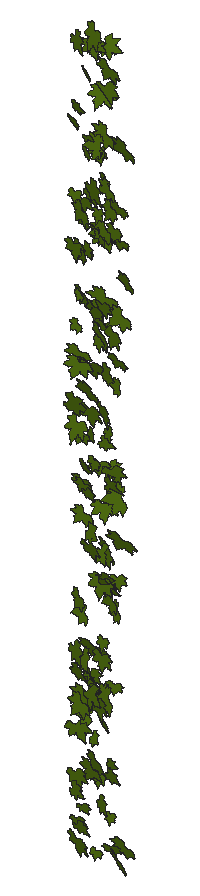
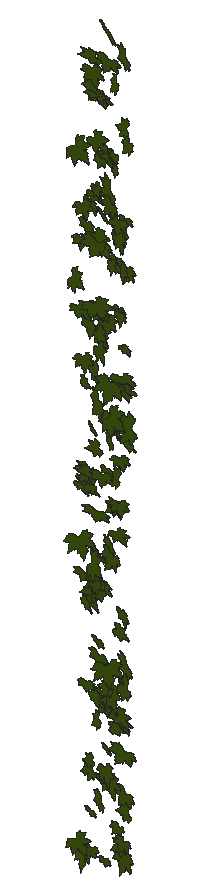
# SketchUp Ruby script. Lengths in inches.
U = 1.inch
M = Sketchup.active_model
def pt(a) = Geom::Point3d.new(a.map { |v| v * U })
def face(e, loops, mat)
  f = e.add_face(loops[0].map { |a| pt(a) })
  loops[1..].each { |l| e.add_face(l.map { |a| pt(a) }).erase! }
  f.material = f.back_material = mat if mat
  f
end
# faces: each face lists its corners as indices into pts; further lists are holes
def faces(e, pts, list, mat = nil) = list.each { |f| face(e, (f[0].is_a?(Array) ? f : [f]).map { |l| l.map { |i| pts[i] } }, mat) }
# xy, xz, yz: faces in a plane at the given z, y or x. An outline is a flat list of corners, or four numbers for a rectangle; further outlines are holes
def ring(l) = l.size == 4 ? [[l[0], l[1]], [l[2], l[1]], [l[2], l[3]], [l[0], l[3]]] : l.each_slice(2).to_a
def flat(e, list, mat, &to3) = list.each { |f| face(e, (f[0].is_a?(Array) ? f : [f]).map { |l| ring(l).map { |u, v| to3.(u, v) } }, mat) }
def xy(e, z, list, mat = nil) = flat(e, list, mat) { |x, y| [x, y, z] }
def xz(e, y, list, mat = nil) = flat(e, list, mat) { |x, z| [x, y, z] }
def yz(e, x, list, mat = nil) = flat(e, list, mat) { |y, z| [x, y, z] }
def lines(e, pts, list) = list.each { |a, b| e.add_line(pt(pts[a]), pt(pts[b])) }
# prism: a flat outline (further loops are holes) pulled along v
def prism(e, loops, v, mat = nil)
  f = face(e, loops, mat); d = Geom::Vector3d.new(v.map { |x| x * U })
  f.pushpull(f.normal.samedirection?(d) ? d.length : -d.length)
end
def box(e, o, s, mat = nil) = prism(e, [[o, [o[0] + s[0], o[1], o[2]], [o[0] + s[0], o[1] + s[1], o[2]], [o[0], o[1] + s[1], o[2]]]], [0, 0, s[2]], mat)
def at(x, y, z, deg = 0) = Geom::Transformation.translation(pt([x, y, z])) * Geom::Transformation.rotation(ORIGIN, Z_AXIS, deg.degrees)
def axes(o, x, y, z) = Geom::Transformation.new([*x, 0, *y, 0, *z, 0, *pt(o).to_a, 1])
def part(name) = M.definitions.add(name)
# library, detail: a bought-in or finely detailed component or shape, given as its bounding box
def library(name, o, s) = part(name).tap { |d| box(d.entities, o, s) }
def detail(e, o, s) = box(e.add_group.entities, o, s)
def put(e, d, t, mat = nil) = e.add_instance(d, t).tap { |i| i.material = mat if mat }
def group(e, t, mat = nil) = e.add_group.tap { |g| g.transformation = t; g.material = mat if mat }.entities
root = M.entities
M.materials.add("[Vegetation Blur 03]").color = [83, 114, 18]
c1 = part("ivy")
xy(c1.entities,0,[[0.782,0,0.786,0,0.787,0.005,0.789,0.009,0.821,0.072,0.875,0.147,1.001,0.272,1.073,0.331,1.137,0.363,1.178,0.379,1.223,0.384,1.272,0.383,1.311,0.374,1.36,0.355,1.399,0.334,1.491,0.285,1.541,0.244,1.583,0.199,1.617,0.15,1.64,0.128,1.662,0.115,1.717,0.105,1.745,0.093,1.784,0.054,1.819,0.057,1.854,0.064,1.882,0.075,1.896,0.074,1.91,0.071,1.937,0.063,1.964,0.053,1.99,0.038,2.016,0.015,2.034,0.002,2.04,0,2.038,0.003,2.036,0.007,2.033,0.038,2.036,0.068,2.045,0.1,2.055,0.116,2.064,0.123,2.077,0.129,2.088,0.129,2.106,0.132,2.118,0.13,2.179,0.132,2.207,0.133,2.225,0.133,2.242,0.138,2.22,0.162,2.207,0.186,2.206,0.213,2.212,0.236,2.228,0.262,2.247,0.274,2.298,0.283,2.355,0.294,2.37,0.296,2.376,0.295,2.377,0.3,2.377,0.303,2.385,0.329,2.411,0.37,2.426,0.392,2.449,0.407,2.511,0.426,2.561,0.444,2.619,0.466,2.589,0.469,2.561,0.476,2.501,0.5,2.449,0.516,2.424,0.523,2.401,0.535,2.377,0.556,2.372,0.568,2.36,0.575,2.268,0.586,2.225,0.592,2.207,0.599,2.194,0.61,2.143,0.65,2.13,0.664,2.122,0.682,2.123,0.7,2.13,0.719,2.148,0.75,2.17,0.781,2.195,0.807,2.221,0.828,2.284,0.874,2.291,0.88,2.288,0.887,2.276,0.9,2.267,0.916,2.265,0.933,2.273,0.967,2.292,1.002,2.313,1.03,2.334,1.054,2.348,1.067,2.358,1.074,2.363,1.076,2.362,1.081,2.35,1.094,2.347,1.11,2.35,1.143,2.359,1.18,2.385,1.254,2.415,1.324,2.448,1.393,2.45,1.4,2.446,1.398,2.44,1.394,2.427,1.383,2.402,1.36,2.376,1.339,2.345,1.324,2.305,1.309,2.282,1.303,2.273,1.306,2.245,1.294,2.212,1.287,2.187,1.291,2.163,1.301,2.142,1.316,2.134,1.327,2.124,1.325,2.09,1.292,2.053,1.259,2.014,1.234,1.973,1.215,1.954,1.21,1.931,1.208,1.909,1.212,1.893,1.22,1.879,1.233,1.872,1.248,1.867,1.281,1.864,1.319,1.821,1.258,1.773,1.197,1.726,1.141,1.698,1.121,1.679,1.116,1.666,1.117,1.647,1.122,1.632,1.129,1.62,1.141,1.617,1.154,1.617,1.219,1.621,1.254,1.623,1.268,1.623,1.281,1.618,1.314,1.606,1.346,1.603,1.375,1.607,1.403,1.603,1.467,1.599,1.499,1.605,1.525,1.614,1.552,1.629,1.577,1.635,1.589,1.629,1.587,1.618,1.582,1.596,1.566,1.581,1.556,1.568,1.552,1.557,1.55,1.545,1.553,1.531,1.562,1.522,1.572,1.504,1.591,1.486,1.611,1.474,1.631,1.457,1.666,1.455,1.684,1.457,1.698,1.452,1.715,1.444,1.728,1.424,1.754,1.419,1.772,1.423,1.786,1.434,1.819,1.444,1.848,1.446,1.855,1.44,1.861,1.43,1.867,1.386,1.904,1.349,1.948,1.326,1.973,1.31,1.995,1.288,2.048,1.284,2.153,1.287,2.254,1.284,2.255,1.282,2.253,1.278,2.247,1.274,2.237,1.266,2.216,1.226,2.125,1.208,2.076,1.184,2.033,1.155,1.984,1.135,1.942,1.111,1.899,1.083,1.861,1.053,1.85,1.059,1.83,1.061,1.809,1.056,1.79,1.049,1.767,1.04,1.749,1.018,1.733,0.994,1.726,0.942,1.734,0.95,1.6875,0.944,1.645,0.932,1.608,0.911,1.585,0.881,1.58,0.854,1.582,0.828,1.588,0.785,1.618,0.773,1.625,0.775,1.614,0.779,1.598,0.796,1.502,0.818,1.402,0.861,1.283,0.882,1.224,0.894,1.174,0.892,1.148,0.886,1.123,0.881,1.107,0.872,1.099,0.849,1.094,0.818,1.092,0.789,1.098,0.762,1.107,0.753,1.113,0.721,1.139,0.698,1.163,0.678,1.194,0.665,1.224,0.628,1.28,0.612,1.312,0.606,1.327,0.606,1.314,0.599,1.282,0.594,1.267,0.581,1.256,0.544,1.245,0.512,1.244,0.473,1.249,0.444,1.256,0.382,1.288,0.339,1.306,0.324,1.316,0.317,1.324,0.309,1.326,0.27,1.314,0.227,1.313,0.185,1.3125,0.152,1.317,0.122,1.328,0.092,1.345,0.073,1.353,0.079,1.338,0.092,1.308,0.117,1.249,0.13,1.215,0.139,1.164,0.147,1.148,0.157,1.136,0.163,1.122,0.174,1.086,0.177,1.067,0.182,1.054,0.186,1.043,0.191,1.038,0.211,1.028,0.237,1.005,0.25,0.974,0.253,0.96,0.25,0.944,0.242,0.914,0.243,0.906,0.249,0.902,0.26,0.894,0.289,0.88,0.307,0.873,0.322,0.862,0.364,0.799,0.403,0.738,0.431,0.709,0.439,0.691,0.441,0.678,0.4375,0.66,0.428,0.645,0.394,0.623,0.303,0.594,0.255,0.581,0.214,0.577,0.179,0.573,0.173,0.568,0.175,0.561,0.167,0.55,0.141,0.523,0.113,0.503,0.077,0.49,0.045,0.486,0.026,0.485,0.019,0.486,0.011,0.483,0,0.471,0.014,0.467,0.044,0.455,0.058,0.447,0.07,0.438,0.097,0.411,0.125,0.394,0.158,0.377,0.174,0.366,0.182,0.359,0.185,0.361,0.242,0.331,0.253,0.316,0.258,0.303,0.262,0.283,0.274,0.278,0.308,0.274,0.341,0.252,0.366,0.226,0.366,0.222,0.37,0.22,0.38,0.221,0.395,0.221,0.425,0.216,0.45,0.207,0.465,0.192,0.473,0.178,0.484,0.15,0.489,0.116,0.483,0.089,0.468,0.058,0.45,0.035,0.435,0.018,0.429,0.011,0.434,0.012,0.438,0.014,0.469,0.019,0.542,0.016,0.581,0.015,0.612,0.027,0.68,0.055,0.696,0.057,0.712,0.052,0.73,0.045,0.741,0.036,0.766,0.014]])
put(root,c1,axes([131.39,173.8,39.79],[0.32765,-0.02489,0.01881],[0.02157,-0.07508,-0.26601],[-0.01455,-0.67173,0.02903]),"[Vegetation Blur 03]")
put(root,c1,axes([131.42,173.8,31.85],[0.50815,0.02983,-0.17456],[-0.21367,-0.02159,-0.41487],[0.01743,-1.13431,0.00331]),"[Vegetation Blur 03]")
put(root,c1,axes([131.75,173.8,33.24],[0.24945,-0.08617,-0.15972],[-0.19859,-0.02674,-0.20432],[-0.02483,-0.6519,0.02949]),"[Vegetation Blur 03]")
put(root,c1,axes([131.27,173.8,43.5625],[0.34754,-0.2147,0.09746],[0.13272,0.06991,-0.29103],[-0.08677,-0.75297,-0.05481]),"[Vegetation Blur 03]")
put(root,c1,axes([132.4375,173.8,30.04],[0.15268,0.21133,-0.48982],[-0.60568,0.18355,-0.11329],[-0.06257,-1.26109,-0.09857]),"[Vegetation Blur 03]")
put(root,c1,axes([131.4,173.8,31.3],[0.55742,0.02012,-0.13001],[-0.15728,-0.13301,-0.4524],[0.0271,-1.18554,0.04855]),"[Vegetation Blur 03]")
put(root,c1,axes([131.15,173.8,37.24],[0.58629,-0.17522,0.04019],[0.04988,0.00183,-0.48347],[-0.08478,-1.21072,-0.00655]),"[Vegetation Blur 03]")
put(root,c1,axes([131.63,173.8,27.5],[0.38921,0.02788,-0.11804],[-0.14492,0.01541,-0.31769],[0.01009,-0.85429,-0.00958]),"[Vegetation Blur 03]")
put(root,c1,axes([131.97,173.8,39.32],[0.36249,-0.1648,-0.3565],[-0.41016,0.32061,-0.3011],[-0.17026,-1.12322,-0.03364]),"[Vegetation Blur 03]")
put(root,c1,axes([131.62,173.8,25.16],[0.40951,0.01971,-0.10583],[-0.13003,0.06915,-0.33309],[-0.00105,-0.88123,-0.0285]),"[Vegetation Blur 03]")
put(root,c1,axes([131.39,173.8,7.37],[0.37849,-0.06704,0.09137],[0.11442,0.06293,-0.30843],[-0.02244,-0.80977,-0.03153]),"[Vegetation Blur 03]")
put(root,c1,axes([131.02,173.8,12.03],[0.53376,0.03726,0.21952],[0.269,0.00727,-0.43585],[0.01776,-1.22992,0.00407]),"[Vegetation Blur 03]")
put(root,c1,axes([131.98,173.8,14.45],[0.42826,-0.11256,-0.35023],[-0.42906,0.04831,-0.35189],[-0.05529,-1.24664,0.01798]),"[Vegetation Blur 03]")
put(root,c1,axes([131.08,173.8,28.28],[0.20202,-0.16973,0.51163],[0.63222,0.07532,-0.16235],[0.00985,-1.35325,-0.07321]),"[Vegetation Blur 03]")
put(root,c1,axes([132.31,173.8,18.72],[0.19822,-0.13225,-0.36337],[-0.44645,0.06503,-0.16594],[-0.0552,-1.0008,0.03723]),"[Vegetation Blur 03]")
put(root,c1,axes([131.39,173.8,8.5],[0.13655,-0.05783,0.35944],[0.43753,-0.10617,-0.1134],[-0.05764,-0.9429,-0.00928]),"[Vegetation Blur 03]")
put(root,c1,axes([131.75,173.8,14.03],[0.51915,-0.17766,-0.225],[-0.28069,-0.03421,-0.42714],[-0.06834,-1.20911,0.04515]),"[Vegetation Blur 03]")
put(root,c1,axes([131.17,173.8,9.74],[0.52125,-0.12471,0.19571],[0.23821,-0.0569,-0.42827],[-0.06661,-1.17932,-0.00003]),"[Vegetation Blur 03]")
put(root,c1,axes([131.91,173.8,23.69],[0.40363,-0.02669,-0.22372],[-0.27442,-0.04788,-0.32887],[0.00236,-1.00289,0.02165]),"[Vegetation Blur 03]")
put(root,c1,axes([131.85,173.8,25.06],[0.38167,-0.01698,-0.15187],[-0.18516,0.0606,-0.31101],[-0.02031,-0.87168,-0.01866]),"[Vegetation Blur 03]")
put(root,c1,axes([131.73,173.8,19.37],[0.45232,-0.27078,-0.13351],[-0.16346,0.04761,-0.38403],[-0.13176,-0.98864,0.01808]),"[Vegetation Blur 03]")
put(root,c1,axes([131.875,173.8,34.86],[0.28246,-0.12607,-0.06429],[-0.08477,-0.04633,-0.23378],[-0.05266,-0.60166,0.03147]),"[Vegetation Blur 03]")
put(root,c1,axes([131.84,173.8,39.18],[0.47471,-0.2198,-0.23723],[-0.27334,0.21714,-0.39597],[-0.14555,-1.12467,-0.03009]),"[Vegetation Blur 03]")
put(root,c1,axes([132.33,173.8,31.25],[0.13027,0.06294,-0.24641],[-0.30303,0.06322,-0.10416],[-0.01626,-0.67369,-0.0328]),"[Vegetation Blur 03]")
put(root,c1,axes([131.27,173.8,6.72],[0.66178,-0.29714,0.00728],[0.02239,0.12543,-0.55031],[-0.14293,-1.35615,-0.0525]),"[Vegetation Blur 03]")
put(root,c1,axes([131.83,173.8,39.5],[0.50423,-0.25138,-0.23976],[-0.28758,0.12452,-0.42338],[-0.1361,-1.1944,0.00632]),"[Vegetation Blur 03]")
put(root,c1,axes([131.65,173.8,43.92],[0.06833,-0.14193,0.31087],[0.38368,-0.0807,-0.06197],[-0.05132,-0.79223,-0.04938]),"[Vegetation Blur 03]")
put(root,c1,axes([131.74,173.8,37.44],[0.499,-0.30069,-0.16614],[-0.19194,0.14146,-0.42426],[-0.16109,-1.09995,-0.00914]),"[Vegetation Blur 03]")
put(root,c1,axes([131.42,173.8,28.24],[0.61381,-0.2023,0.00115],[-0.01893,-0.26118,-0.49641],[-0.09648,-1.23581,0.10472]),"[Vegetation Blur 03]")
put(root,c1,axes([131.78,173.8,35.02],[0.4623,-0.23108,-0.11744],[-0.13279,0.12742,-0.38762],[-0.12523,-0.98816,-0.02252]),"[Vegetation Blur 03]")
put(root,c1,axes([131.5625,173.8,39.6],[0.49002,-0.06773,0.03255],[0.04203,0.06603,-0.39982],[-0.03013,-1.00954,-0.02833]),"[Vegetation Blur 03]")
put(root,c1,axes([131.43,173.8,14.87],[0.2552,-0.21443,0.36363],[0.45118,-0.05704,-0.2162],[-0.07626,-1.05507,-0.06222]),"[Vegetation Blur 03]")
put(root,c1,axes([131.3,173.8,16.1],[0.40591,-0.18014,0.3374],[0.39655,-0.24525,-0.33836],[-0.14603,-1.16675,0.01903]),"[Vegetation Blur 03]")
put(root,c1,axes([131.77,173.8,8.02],[0.2717,-0.01326,0.11926],[0.14597,0.06528,-0.22036],[0.00938,-0.63148,-0.02528]),"[Vegetation Blur 03]")
put(root,c1,axes([131.55,173.8,6.9],[0.29257,-0.13243,0.26003],[0.3239,0.04481,-0.23915],[-0.02726,-0.88901,-0.05079]),"[Vegetation Blur 03]")
put(root,c1,axes([131.42,173.8,47.55],[0.32606,-0.15993,0.37004],[0.43652,-0.25327,-0.27342],[-0.14515,-1.12098,0.00898]),"[Vegetation Blur 03]")
put(root,c1,axes([132.34,173.8,15.5625],[0.44681,-0.13861,-0.40686],[-0.47518,0.33403,-0.36549],[-0.1651,-1.33648,-0.04915]),"[Vegetation Blur 03]")
put(root,c1,axes([132.76,173.8,13.41],[0.05855,-0.11186,-0.32035],[-0.39567,-0.06136,-0.0448],[0.02177,-0.81436,0.04738]),"[Vegetation Blur 03]")
put(root,c1,axes([132.01,173.8,16.84],[0.5883,0.12569,-0.22776],[-0.28567,0.25569,-0.4693],[0.00068,-1.31528,-0.113]),"[Vegetation Blur 03]")
put(root,c1,axes([132.23,173.8,42.33],[0.2858,-0.16556,-0.09391],[-0.1058,0.0991,-0.24194],[-0.0923,-0.62621,-0.01346]),"[Vegetation Blur 03]")
put(root,c1,axes([131.67,173.8,31.23],[0.67545,-0.01499,0.0047],[0.00705,0.26519,-0.54115],[-0.00605,-1.36446,-0.10523]),"[Vegetation Blur 03]")
put(root,c1,axes([132.31,173.8,37.39],[0.30779,-0.16022,-0.12096],[-0.12595,0.19898,-0.2549],[-0.11031,-0.67423,-0.04648]),"[Vegetation Blur 03]")
put(root,c1,axes([131.82,173.8,15.51],[0.22572,0.02556,0.3673],[0.42622,-0.34586,-0.17068],[-0.14503,-0.97663,0.07006]),"[Vegetation Blur 03]")
put(root,c1,axes([132.1,173.8,42.75],[0.27595,-0.07999,0.10883],[0.13684,0.05207,-0.2251],[-0.02378,-0.62852,-0.0325]),"[Vegetation Blur 03]")
put(root,c1,axes([132.26,173.8,10.78],[0.5571,-0.15804,-0.2532],[-0.30286,0.14883,-0.45846],[-0.10211,-1.30372,-0.02164]),"[Vegetation Blur 03]")
put(root,c1,axes([131.99,173.8,36.92],[0.26922,-0.1042,0.25304],[0.30661,-0.09593,-0.2235],[-0.06845,-0.83952,-0.00587]),"[Vegetation Blur 03]")
put(root,c1,axes([132.17,173.8,25.57],[0.07402,-0.1812,0.31745],[0.39109,-0.12634,-0.07209],[-0.07805,-0.80492,-0.06015]),"[Vegetation Blur 03]")
put(root,c1,axes([132.11,173.8,46.38],[0.3403,-0.29163,0.09942],[0.13762,0.03874,-0.29588],[-0.12643,-0.74278,-0.05447]),"[Vegetation Blur 03]")
put(root,c1,axes([132.08,173.8,24.4],[0.28875,-0.1223,0.18363],[0.229,0.01809,-0.23796],[-0.04139,-0.75306,-0.03554]),"[Vegetation Blur 03]")
put(root,c1,axes([131.86,173.8,28.96],[0.63148,-0.16792,0.0994],[0.12538,0.04433,-0.51879],[-0.07597,-1.32267,-0.03001]),"[Vegetation Blur 03]")
put(root,c1,axes([132.12,173.8,14.93],[0.31712,0.01449,0.22059],[0.2693,0.0595,-0.25849],[0.0241,-0.85537,-0.01424]),"[Vegetation Blur 03]")
put(root,c1,axes([131.97,173.8,47.6875],[0.52799,0.03971,0.1403],[0.17249,-0.03446,-0.43082],[0.01316,-1.14211,0.01788]),"[Vegetation Blur 03]")
put(root,c1,axes([132.26,173.8,34.47],[0.55471,-0.15442,-0.09413],[-0.10485,0.16405,-0.45388],[-0.08911,-1.1543,-0.05191]),"[Vegetation Blur 03]")
put(root,c1,axes([131.98,173.8,21.86],[0.52924,-0.21641,0.13482],[0.17446,0.07604,-0.43695],[-0.08896,-1.13835,-0.05482]),"[Vegetation Blur 03]")
put(root,c1,axes([132.57,173.8,11.23],[0.48731,-0.17978,-0.24983],[-0.29064,0.21865,-0.40235],[-0.12987,-1.16387,-0.037]),"[Vegetation Blur 03]")
put(root,c1,axes([132.29,173.8,22.02],[0.07963,0.08394,0.36792],[0.43963,-0.2386,-0.05481],[-0.10777,-0.91131,0.04824]),"[Vegetation Blur 03]")
put(root,c1,axes([132.97,173.8,38.43],[0.27575,-0.07071,-0.32237],[-0.38727,0.16418,-0.22631],[-0.08498,-0.9776,-0.01469]),"[Vegetation Blur 03]")
put(root,c1,axes([132.84,173.8,42.93],[0.3287,-0.1611,-0.24597],[-0.30329,0.03864,-0.27395],[-0.07054,-0.91688,0.03167]),"[Vegetation Blur 03]")
put(root,c1,axes([132.14,173.8,39.98],[0.42324,-0.15513,0.17492],[0.21736,0.00516,-0.3496],[-0.06611,-0.97622,-0.02964]),"[Vegetation Blur 03]")
put(root,c1,axes([133.29,173.8,43.27],[0.20332,-0.17652,-0.4378],[-0.54125,0.03497,-0.16965],[-0.04646,-1.17997,0.06046]),"[Vegetation Blur 03]")
put(root,c1,axes([132.52,173.8,14.13],[0.08923,-0.0651,0.22881],[0.28147,0.0622,-0.07033],[0.01942,-0.60224,-0.032]),"[Vegetation Blur 03]")
put(root,c1,axes([132.56,173.8,26.42],[0.35274,-0.11868,-0.02991],[-0.03922,-0.02703,-0.29129],[-0.05595,-0.72928,0.01566]),"[Vegetation Blur 03]")
put(root,c1,axes([132.55,173.8,11.58],[0.08406,0.07505,0.23958],[0.28752,-0.16835,-0.0589],[-0.06954,-0.60538,0.04608]),"[Vegetation Blur 03]")
put(root,c1,axes([132.44,173.8,27.51],[0.18332,-0.13201,0.23981],[0.28131,-0.17522,-0.15841],[-0.10639,-0.6908,-0.00565]),"[Vegetation Blur 03]")
put(root,c1,axes([133.55,173.8,22.12],[0.10735,0.13666,-0.49936],[-0.59338,0.3622,-0.06937],[-0.16335,-1.22594,-0.07616]),"[Vegetation Blur 03]")
put(root,c1,axes([132.66,173.8,6.17],[0.29298,-0.03076,-0.00517],[-0.00747,-0.046,-0.2387],[-0.01442,-0.60127,0.01853]),"[Vegetation Blur 03]")
put(root,c1,axes([133.12,173.8,33.08],[0.29122,-0.09132,-0.34949],[-0.40801,0.28097,-0.238],[-0.13739,-1.02797,-0.034]),"[Vegetation Blur 03]")
put(root,c1,axes([133.26,173.8,33.86],[0.15958,-0.02123,-0.31626],[-0.37905,0.17205,-0.12921],[-0.08118,-0.84504,-0.01836]),"[Vegetation Blur 03]")
put(root,c1,axes([132.14,173.8,13.62],[0.16056,0.04012,0.53459],[0.63688,-0.33645,-0.12344],[-0.15436,-1.34643,0.04677]),"[Vegetation Blur 03]")
put(root,c1,axes([132.49,173.8,26.21],[0.45127,0.0715,0.00789],[0.01018,-0.0128,-0.36935],[0.0346,-0.92876,0.0057]),"[Vegetation Blur 03]")
put(root,c1,axes([132.98,173.8,35.38],[0.53259,0.07407,-0.33493],[-0.4092,-0.06459,-0.43565],[0.04766,-1.38209,0.00241]),"[Vegetation Blur 03]")
put(root,c1,axes([133.35,173.8,43.9375],[0.36403,-0.06267,-0.40957],[-0.5016,0.04126,-0.29795],[-0.03412,-1.27511,0.01049]),"[Vegetation Blur 03]")
put(root,c1,axes([133.33,173.8,41.21],[0.19632,-0.0358,-0.23719],[-0.2774,0.19596,-0.15758],[-0.08838,-0.69459,-0.03223]),"[Vegetation Blur 03]")
put(root,c1,axes([132.84,173.8,42.38],[0.31483,-0.06922,0.03461],[0.04453,0.03834,-0.25772],[-0.03078,-0.65259,-0.01881]),"[Vegetation Blur 03]")
put(root,c1,axes([133.11,173.8,38.875],[0.46325,-0.03451,-0.29794],[-0.36488,0.02419,-0.37832],[-0.02045,-1.21347,0.00093]),"[Vegetation Blur 03]")
put(root,c1,axes([132.59,173.8,49],[0.61554,-0.40401,-0.01131],[-0.04771,-0.21545,-0.519],[-0.19095,-1.24853,0.09322]),"[Vegetation Blur 03]")
put(root,c1,axes([132.81,173.8,33.5],[0.58606,-0.32249,-0.17371],[-0.19607,0.18401,-0.49434],[-0.17725,-1.2698,-0.02752]),"[Vegetation Blur 03]")
put(root,c1,axes([132.25,173.8,40.22],[0.41734,-0.25524,0.42347],[0.50918,-0.21404,-0.35453],[-0.15923,-1.35344,-0.02379]),"[Vegetation Blur 03]")
put(root,c1,axes([132.88,173.8,10.16],[0.34421,-0.10508,0.04416],[0.04441,-0.1326,-0.28022],[-0.05969,-0.70465,0.04615]),"[Vegetation Blur 03]")
put(root,c1,axes([132.84,173.8,39.36],[0.35292,-0.17211,0.08002],[0.07901,-0.17569,-0.29156],[-0.10181,-0.73298,0.0511]),"[Vegetation Blur 03]")
put(root,c1,axes([132.81,173.8,32.67],[0.3385,-0.12078,0.12895],[0.14584,-0.15588,-0.27795],[-0.08451,-0.75275,0.03687]),"[Vegetation Blur 03]")
put(root,c1,axes([132.6,173.8,20.47],[0.64834,-0.11558,0.00243],[-0.00125,-0.10055,-0.52962],[-0.05623,-1.33037,0.03982]),"[Vegetation Blur 03]")
put(root,c1,axes([133.59,173.8,41.03],[0.26205,-0.06963,-0.34462],[-0.42004,0.08964,-0.2156],[-0.05487,-1.01871,0.00458]),"[Vegetation Blur 03]")
put(root,c1,axes([132.8125,173.8,45.82],[0.58164,-0.02914,-0.08506],[-0.10504,-0.22356,-0.46637],[0.00547,-1.19524,0.0893]),"[Vegetation Blur 03]")
put(root,c1,axes([133.73,173.8,15.02],[0.29249,-0.26424,-0.46367],[-0.56799,0.1604,-0.25303],[-0.12902,-1.30512,0.06278]),"[Vegetation Blur 03]")
put(root,c1,axes([133.12,173.8,20.43],[0.29824,-0.02143,-0.02343],[-0.02665,0.10046,-0.24043],[-0.01491,-0.60833,-0.03888]),"[Vegetation Blur 03]")
put(root,c1,axes([132.47,173.8,38.03],[0.60611,0.08882,0.16972],[0.20851,-0.00255,-0.49577],[0.04043,-1.31863,0.01239]),"[Vegetation Blur 03]")
put(root,c1,axes([132.64,173.8,24.07],[0.5345,0.11261,0.12686],[0.16236,-0.17388,-0.43135],[0.02823,-1.13219,0.07887]),"[Vegetation Blur 03]")
put(root,c1,axes([132.8125,173.8,34.49],[0.44672,-0.11391,0.09884],[0.12385,0.0351,-0.3665],[-0.0489,-0.9518,-0.02535]),"[Vegetation Blur 03]")
put(root,c1,axes([133.07,173.8,17.28],[0.33589,-0.10606,0.03492],[0.03467,-0.10992,-0.27466],[-0.05731,-0.68805,0.03849]),"[Vegetation Blur 03]")
put(root,c1,axes([132.54,173.8,14.03],[0.57796,-0.29472,0.19025],[0.2281,-0.10009,-0.48593],[-0.15109,-1.27852,-0.00582]),"[Vegetation Blur 03]")
put(root,c1,axes([132.97,173.8,42.2],[0.24496,-0.07431,0.21292],[0.23492,-0.26987,-0.19483],[-0.11909,-0.6852,0.05364]),"[Vegetation Blur 03]")
put(root,c1,axes([132.76,173.8,16.54],[0.56428,-0.16916,0.04285],[0.04868,-0.06133,-0.46503],[-0.08453,-1.16458,0.01826]),"[Vegetation Blur 03]")
put(root,c1,axes([132.81,173.8,21.47],[0.29882,0.02623,0.28715],[0.33985,-0.26962,-0.23169],[-0.09199,-0.91085,0.07685]),"[Vegetation Blur 03]")
put(root,c1,axes([133.03,173.8,26.99],[0.12471,-0.00455,0.29508],[0.36083,0.05141,-0.10146],[0.0229,-0.78534,-0.00835]),"[Vegetation Blur 03]")
put(root,c1,axes([133.1875,173.8,47.26],[0.56003,-0.11483,-0.22477],[-0.26984,0.13286,-0.4585],[-0.07841,-1.27735,-0.02748]),"[Vegetation Blur 03]")
put(root,c1,axes([132.82,173.8,20.17],[0.35675,-0.1356,0.28151],[0.35114,0.1247,-0.28695],[-0.00453,-1.0135,-0.07297]),"[Vegetation Blur 03]")
put(root,c1,axes([133.75,173.8,19.94],[0.31943,-0.14813,-0.35105],[-0.42397,0.15166,-0.26703],[-0.10221,-1.09204,0.01053]),"[Vegetation Blur 03]")
put(root,c1,axes([132.95,173.8,8.52],[0.23742,-0.1267,0.33587],[0.39552,-0.23419,-0.20013],[-0.12927,-0.94922,0.00454]),"[Vegetation Blur 03]")
put(root,c1,axes([133.07,173.8,47.25],[0.0857,0.17777,0.39101],[0.48593,0.02942,-0.07304],[0.02949,-1.0011,0.06729]),"[Vegetation Blur 03]")
put(root,c1,axes([133.16,173.8,12.93],[0.26661,-0.22568,0.1584],[0.20153,-0.02212,-0.2309],[-0.09528,-0.67823,-0.04518]),"[Vegetation Blur 03]")
put(root,c1,axes([132.84,173.8,19.58],[0.27593,-0.17427,0.39331],[0.48854,0.16147,-0.21704],[0.02723,-1.13128,-0.09157]),"[Vegetation Blur 03]")
put(root,c1,axes([133.25,173.8,6.52],[0.36983,0.02306,0.04655],[0.05424,0.13467,-0.29755],[0.02088,-0.75816,-0.05144]),"[Vegetation Blur 03]")
put(root,c1,axes([132.77,173.8,45.69],[0.56787,-0.08069,0.24242],[0.2938,-0.10677,-0.464],[-0.05873,-1.31444,0.02281]),"[Vegetation Blur 03]")
put(root,c1,axes([133.29,173.8,30.59],[0.06006,-0.04189,0.40073],[0.47866,-0.22553,-0.0515],[-0.11129,-0.99263,-0.00521]),"[Vegetation Blur 03]")
put(root,c1,axes([133.1875,173.8,21.59],[0.33061,-0.13828,0.23143],[0.27228,-0.16795,-0.27487],[-0.10387,-0.88042,0.01609]),"[Vegetation Blur 03]")
put(root,c1,axes([133.41,173.8,27.97],[0.2323,-0.07315,0.16912],[0.19295,-0.17827,-0.18866],[-0.08352,-0.61528,0.03456]),"[Vegetation Blur 03]")
put(root,c1,axes([132.98,173.8,29.38],[0.56286,-0.41503,0.17137],[0.21267,-0.05627,-0.48669],[-0.19885,-1.23496,-0.03542]),"[Vegetation Blur 03]")
put(root,c1,axes([133.52,173.8,8.3],[0.28663,-0.07213,0.05383],[0.05877,-0.11436,-0.23255],[-0.04609,-0.59433,0.03821]),"[Vegetation Blur 03]")
put(root,c1,axes([133.58,173.8,40.08],[0.46163,-0.2581,-0.13642],[-0.17424,-0.01487,-0.3883],[-0.11538,-1.01019,0.04057]),"[Vegetation Blur 03]")
put(root,c1,axes([133.46,173.8,25.63],[0.07333,0.12212,0.31359],[0.38829,0.01811,-0.06159],[0.01986,-0.80476,0.0462]),"[Vegetation Blur 03]")
put(root,c1,axes([133.56,173.8,10.65],[0.09053,-0.05831,0.23092],[0.28382,-0.01925,-0.07488],[-0.01758,-0.61103,-0.01968]),"[Vegetation Blur 03]")
put(root,c1,axes([133.54,173.8,15.08],[0.35798,0.03491,0.00358],[0.00487,-0.0205,-0.29237],[0.01684,-0.73641,0.00831]),"[Vegetation Blur 03]")
put(root,c1,axes([133.73,173.8,32.12],[0.41941,-0.00434,-0.1684],[-0.2031,0.16133,-0.33757],[-0.03648,-0.94822,-0.05667]),"[Vegetation Blur 03]")
put(root,c1,axes([133.14,173.8,25.9],[0.48195,0.00963,0.21143],[0.25864,0.04977,-0.39304],[0.01557,-1.12486,-0.01558]),"[Vegetation Blur 03]")
put(root,c1,axes([133.82,173.8,40.09],[0.40291,0.01111,-0.21009],[-0.25613,0.11786,-0.3262],[-0.02632,-0.9768,-0.04175]),"[Vegetation Blur 03]")
put(root,c1,axes([134.34,173.8,30.88],[0.08976,-0.09939,-0.28739],[-0.34963,0.10974,-0.07871],[-0.06393,-0.7397,0.02694]),"[Vegetation Blur 03]")
put(root,c1,axes([134.35,173.8,43.4],[0.2991,0.11532,-0.48246],[-0.59082,0.19391,-0.23668],[-0.05934,-1.34945,-0.07524]),"[Vegetation Blur 03]")
put(root,c1,axes([133.72,173.8,22.99],[0.56725,0.10726,-0.27566],[-0.34171,0.20149,-0.45603],[-0.00596,-1.34353,-0.0904]),"[Vegetation Blur 03]")
put(root,c1,axes([134.18,173.8,19.48],[0.25494,-0.21897,-0.29058],[-0.35433,0.12452,-0.22182],[-0.11199,-0.89248,0.04035]),"[Vegetation Blur 03]")
put(root,c1,axes([133.42,173.8,10.08],[0.21568,-0.13397,0.30172],[0.37321,-0.01782,-0.17894],[-0.04036,-0.88058,-0.04228]),"[Vegetation Blur 03]")
put(root,c1,axes([133.6,173.8,38.82],[0.45457,-0.14322,-0.01986],[-0.02603,-0.01905,-0.37516],[-0.06898,-0.93657,0.01067]),"[Vegetation Blur 03]")
put(root,c1,axes([134.23,173.8,7.27],[0.36107,0.086,-0.36328],[-0.44668,0.11955,-0.29126],[-0.01905,-1.17336,-0.0563]),"[Vegetation Blur 03]")
put(root,c1,axes([133.47,173.8,24.8],[0.10325,-0.14377,0.42811],[0.52829,-0.03594,-0.08677],[-0.03077,-1.09956,-0.05314]),"[Vegetation Blur 03]")
put(root,c1,axes([133.53,173.8,33.7],[0.59158,-0.31026,-0.0564],[-0.07139,-0.00087,-0.49803],[-0.1497,-1.22563,0.01463]),"[Vegetation Blur 03]")
put(root,c1,axes([133.76,173.8,6.52],[0.54071,-0.2448,-0.19934],[-0.20803,0.34691,-0.44288],[-0.17473,-1.17061,-0.08956]),"[Vegetation Blur 03]")
put(root,c1,axes([134.52,173.8,25.6875],[0.30037,-0.23448,-0.48095],[-0.59958,-0.05449,-0.24524],[-0.02777,-1.36002,0.09275]),"[Vegetation Blur 03]")
put(root,c1,axes([133.83,173.8,38.13],[0.37713,0.02521,-0.05482],[-0.06814,0.09104,-0.30568],[0.00422,-0.78299,-0.03731]),"[Vegetation Blur 03]")
put(root,c1,axes([134.13,173.8,34.76],[0.44525,-0.05596,-0.30949],[-0.38019,-0.06333,-0.36251],[-0.0007,-1.20185,0.03351]),"[Vegetation Blur 03]")
put(root,c1,axes([134.71,173.8,36.39],[0.11247,0.10768,-0.41349],[-0.50254,0.19726,-0.08297],[-0.08291,-1.04957,-0.05801]),"[Vegetation Blur 03]")
put(root,c1,axes([133.66,173.8,20.58],[0.38704,0.02073,0.09682],[0.11906,-0.06304,-0.31489],[0.00062,-0.83064,0.02631]),"[Vegetation Blur 03]")
